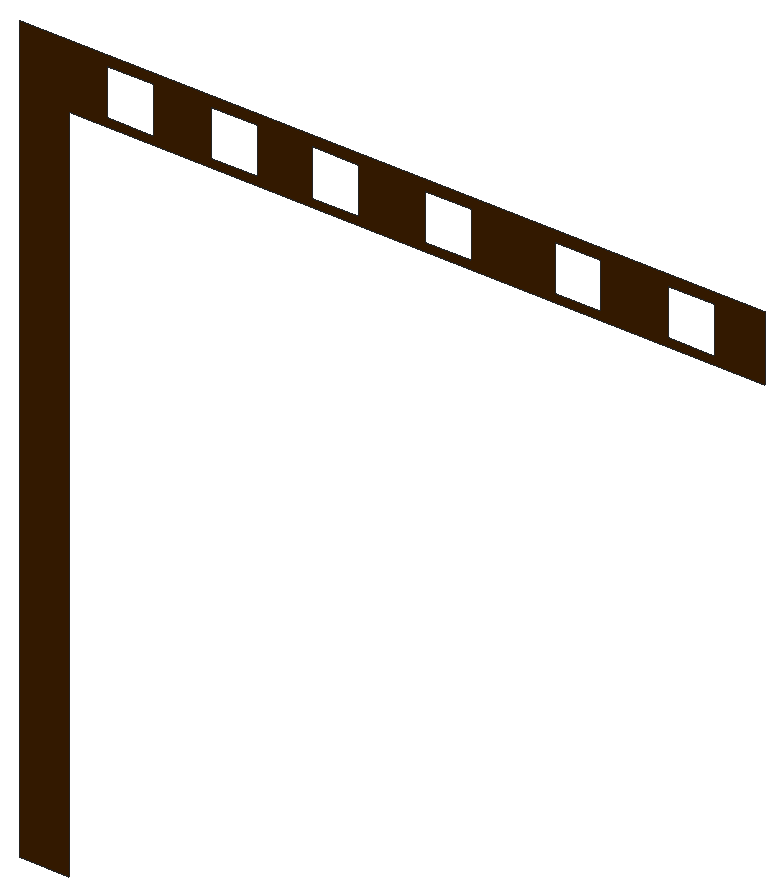
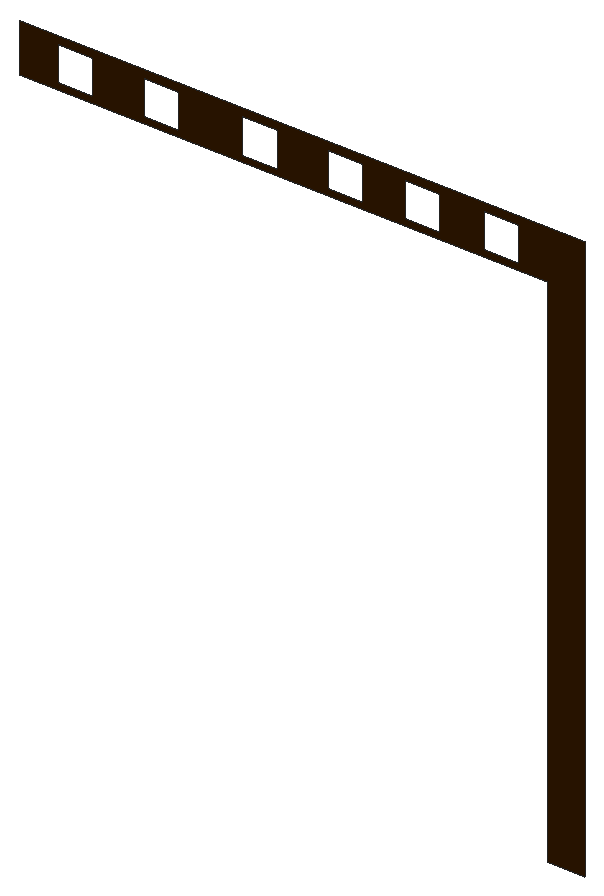
# SketchUp Ruby script. Lengths in inches.
U = 1.inch
M = Sketchup.active_model
def pt(a) = Geom::Point3d.new(a.map { |v| v * U })
def face(e, loops, mat)
  f = e.add_face(loops[0].map { |a| pt(a) })
  loops[1..].each { |l| e.add_face(l.map { |a| pt(a) }).erase! }
  f.material = f.back_material = mat if mat
  f
end
# faces: each face lists its corners as indices into pts; further lists are holes
def faces(e, pts, list, mat = nil) = list.each { |f| face(e, (f[0].is_a?(Array) ? f : [f]).map { |l| l.map { |i| pts[i] } }, mat) }
# xy, xz, yz: faces in a plane at the given z, y or x. An outline is a flat list of corners, or four numbers for a rectangle; further outlines are holes
def ring(l) = l.size == 4 ? [[l[0], l[1]], [l[2], l[1]], [l[2], l[3]], [l[0], l[3]]] : l.each_slice(2).to_a
def flat(e, list, mat, &to3) = list.each { |f| face(e, (f[0].is_a?(Array) ? f : [f]).map { |l| ring(l).map { |u, v| to3.(u, v) } }, mat) }
def xy(e, z, list, mat = nil) = flat(e, list, mat) { |x, y| [x, y, z] }
def xz(e, y, list, mat = nil) = flat(e, list, mat) { |x, z| [x, y, z] }
def yz(e, x, list, mat = nil) = flat(e, list, mat) { |y, z| [x, y, z] }
def lines(e, pts, list) = list.each { |a, b| e.add_line(pt(pts[a]), pt(pts[b])) }
# prism: a flat outline (further loops are holes) pulled along v
def prism(e, loops, v, mat = nil)
  f = face(e, loops, mat); d = Geom::Vector3d.new(v.map { |x| x * U })
  f.pushpull(f.normal.samedirection?(d) ? d.length : -d.length)
end
def box(e, o, s, mat = nil) = prism(e, [[o, [o[0] + s[0], o[1], o[2]], [o[0] + s[0], o[1] + s[1], o[2]], [o[0], o[1] + s[1], o[2]]]], [0, 0, s[2]], mat)
def at(x, y, z, deg = 0) = Geom::Transformation.translation(pt([x, y, z])) * Geom::Transformation.rotation(ORIGIN, Z_AXIS, deg.degrees)
def axes(o, x, y, z) = Geom::Transformation.new([*x, 0, *y, 0, *z, 0, *pt(o).to_a, 1])
def part(name) = M.definitions.add(name)
# library, detail: a bought-in or finely detailed component or shape, given as its bounding box
def library(name, o, s) = part(name).tap { |d| box(d.entities, o, s) }
def detail(e, o, s) = box(e.add_group.entities, o, s)
def put(e, d, t, mat = nil) = e.add_instance(d, t).tap { |i| i.material = mat if mat }
def group(e, t, mat = nil) = e.add_group.tap { |g| g.transformation = t; g.material = mat if mat }.entities
root = M.entities
M.materials.add("[Color C08]").color = [63, 31, 0]
xz(root,210.73,[[[168.19,137.875,176.75,137.875,176.75,257.875,298.6,257.875,298.6,269.25,168.19,269.25],[183.39,259.25,191.57,267.44],[281.76,259.25,289.95,267.44],[201.64,259.25,209.82,267.44],[261.82,259.25,270.01,267.44],[219.32,259.25,227.51,267.44],[239.14,259.25,247.32,267.44]]],"[Color C08]")
